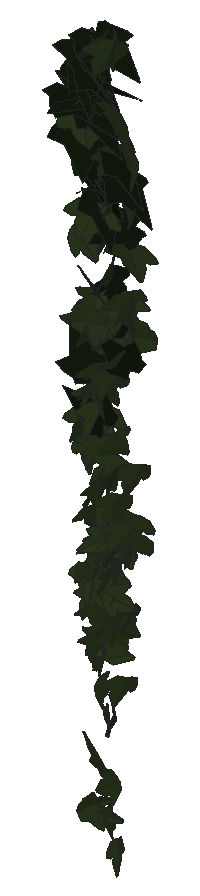
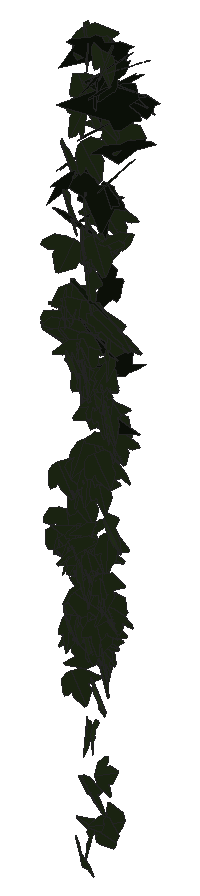
# SketchUp Ruby script. Lengths in inches.
U = 1.inch
M = Sketchup.active_model
def pt(a) = Geom::Point3d.new(a.map { |v| v * U })
def face(e, loops, mat)
  f = e.add_face(loops[0].map { |a| pt(a) })
  loops[1..].each { |l| e.add_face(l.map { |a| pt(a) }).erase! }
  f.material = f.back_material = mat if mat
  f
end
# faces: each face lists its corners as indices into pts; further lists are holes
def faces(e, pts, list, mat = nil) = list.each { |f| face(e, (f[0].is_a?(Array) ? f : [f]).map { |l| l.map { |i| pts[i] } }, mat) }
# xy, xz, yz: faces in a plane at the given z, y or x. An outline is a flat list of corners, or four numbers for a rectangle; further outlines are holes
def ring(l) = l.size == 4 ? [[l[0], l[1]], [l[2], l[1]], [l[2], l[3]], [l[0], l[3]]] : l.each_slice(2).to_a
def flat(e, list, mat, &to3) = list.each { |f| face(e, (f[0].is_a?(Array) ? f : [f]).map { |l| ring(l).map { |u, v| to3.(u, v) } }, mat) }
def xy(e, z, list, mat = nil) = flat(e, list, mat) { |x, y| [x, y, z] }
def xz(e, y, list, mat = nil) = flat(e, list, mat) { |x, z| [x, y, z] }
def yz(e, x, list, mat = nil) = flat(e, list, mat) { |y, z| [x, y, z] }
def lines(e, pts, list) = list.each { |a, b| e.add_line(pt(pts[a]), pt(pts[b])) }
# prism: a flat outline (further loops are holes) pulled along v
def prism(e, loops, v, mat = nil)
  f = face(e, loops, mat); d = Geom::Vector3d.new(v.map { |x| x * U })
  f.pushpull(f.normal.samedirection?(d) ? d.length : -d.length)
end
def box(e, o, s, mat = nil) = prism(e, [[o, [o[0] + s[0], o[1], o[2]], [o[0] + s[0], o[1] + s[1], o[2]], [o[0], o[1] + s[1], o[2]]]], [0, 0, s[2]], mat)
def at(x, y, z, deg = 0) = Geom::Transformation.translation(pt([x, y, z])) * Geom::Transformation.rotation(ORIGIN, Z_AXIS, deg.degrees)
def axes(o, x, y, z) = Geom::Transformation.new([*x, 0, *y, 0, *z, 0, *pt(o).to_a, 1])
def part(name) = M.definitions.add(name)
# library, detail: a bought-in or finely detailed component or shape, given as its bounding box
def library(name, o, s) = part(name).tap { |d| box(d.entities, o, s) }
def detail(e, o, s) = box(e.add_group.entities, o, s)
def put(e, d, t, mat = nil) = e.add_instance(d, t).tap { |i| i.material = mat if mat }
def group(e, t, mat = nil) = e.add_group.tap { |g| g.transformation = t; g.material = mat if mat }.entities
root = M.entities
M.materials.add("1026 AP 7946 SUNNY SIDE UP").color = [254, 231, 186]
M.materials.add("efeu1").color = [18, 25, 13]
M.materials.add("efeu2").color = [43, 57, 29]
c1 = part("ivyleaf_10")
p = [[0,0.5,-0.03],[-0.0625,2.02,-0.43],[-0.19,2.01,-0.46],[-0.54,1.05,-0.29],[-0.52,0.625,-0.18],[-0.83,0.76,-0.28],
  [-1.16,0.64,-0.33],[-1.15,0.33,-0.24],[-0.77,-0.39,0.02],[-0.3,-0.51,0.16],[0.04,-0.48,0.23],[-0.02,2.01,-0.4375],
  [-0.06,2.01,-0.43],[0.04,-0.49,0.23],[0.67,-0.49,0.14],[1.38,0.36,-0.2],[1.375,0.51,-0.24],[0.81,0.65,-0.19],
  [0.62,0.59,-0.15],[0.6,1.09,-0.28],[0.5,1.23,-0.31]]
faces(c1.entities,p,[[0,1,2,3,4,5,6,7,8,9,10],[11,12,0,13,14,15,16,17,18,19,20]],"efeu2")
c2 = part("ivyleaf_9")
p = [[1.54,2.16,1.25],[1.36,2.04,1.19],[-0.21,0.99,0.68],[-0.71,1.11,0.82],[-0.85,0.86,0.67],[-0.8,0.17,0.21],
  [-0.9,-0.01,0.1],[-0.67,-0.16,-0.02],[-0.08,-0.08,-0.05],[-0.03,-0.6,-0.4],[0.65,-0.88,-0.66],[0.83,-0.6,-0.49],
  [1.29,-0.42,-0.43],[1.8125,-0.07,-0.26],[1.21,0.44,0.15]]
faces(c2.entities,p,[[0,1,2,3,4,5,6,7,8,9,10,11,12,13,14]],"efeu1")
put(root,c1,axes([97.41,212.91,259.63],[0.10949,-0.19734,0.03462],[0.00095,-0.03655,-0.21548],[0.31507,0.06869,-0.01138]),"1026 AP 7946 SUNNY SIDE UP")
put(root,c2,axes([97.3125,212.78,265.79],[-0.1247,-0.23157,-0.03696],[0.03509,0.02884,-0.25171],[0.36648,-0.08156,0.01152]),"1026 AP 7946 SUNNY SIDE UP")
put(root,c1,axes([97.43,212.875,261.5],[0.0398,-0.22079,-0.03862],[-0.00634,0.03601,-0.22874],[0.35176,0.02563,0.00025]),"1026 AP 7946 SUNNY SIDE UP")
put(root,c2,axes([97.1,212.91,266.58],[0.33752,-0.03414,0.13387],[0.21069,0.03213,-0.21881],[0.01909,0.24896,0.0481]),"1026 AP 7946 SUNNY SIDE UP")
put(root,c2,axes([97.38,212.9,267.02],[-0.18909,-0.20027,0.10554],[0.00393,-0.11857,-0.23388],[0.35451,-0.10551,0.05889]),"1026 AP 7946 SUNNY SIDE UP")
put(root,c1,axes([97.36,212.92,258.26],[0.31557,-0.04478,0.0197],[0.02354,-0.02155,-0.21118],[0.07301,0.20047,-0.01706]),"1026 AP 7946 SUNNY SIDE UP")
put(root,c1,axes([97.43,212.97,261.54],[0.10388,-0.20513,-0.06291],[-0.00085,0.06254,-0.22088],[0.33602,0.06357,0.01889]),"1026 AP 7946 SUNNY SIDE UP")
put(root,c1,axes([97.42,212.91,259.36],[-0.09153,-0.1926,-0.0574],[0.03273,0.05075,-0.20692],[0.31308,-0.06161,0.00485]),"1026 AP 7946 SUNNY SIDE UP")
put(root,c2,axes([97.58,212.73,266.62],[-0.36277,-0.04896,0.03114],[-0.04029,-0.02881,-0.23387],[0.08849,-0.21383,0.02119]),"1026 AP 7946 SUNNY SIDE UP")
put(root,c1,axes([97.44,212.99,258.75],[-0.08302,-0.19748,-0.02475],[0.02284,0.0198,-0.21027],[0.31176,-0.05404,0.00882]),"1026 AP 7946 SUNNY SIDE UP")
put(root,c1,axes([97.43,212.82,262.5],[0.02247,-0.20885,-0.10627],[0.03565,0.10293,-0.2133],[0.3637,0.00282,0.02747]),"1026 AP 7946 SUNNY SIDE UP")
put(root,c1,axes([97.37,212.86,258.4],[-0.07173,-0.16061,-0.12519],[0.12446,0.0993,-0.16648],[0.29027,-0.08227,0.04044]),"1026 AP 7946 SUNNY SIDE UP")
put(root,c1,axes([97.58,212.9,262.92],[0.25928,-0.04659,-0.15665],[-0.22743,0.04621,-0.17621],[0.103,0.21931,0.00525]),"1026 AP 7946 SUNNY SIDE UP")
put(root,c1,axes([97.68,212.7,262.68],[0.13861,-0.05263,-0.2141],[-0.32312,0.06301,-0.10043],[0.13429,0.20595,-0.02066]),"1026 AP 7946 SUNNY SIDE UP")
put(root,c1,axes([97.35,212.73,266.0625],[0.3438,0.11325,0.03898],[0.0364,0.033,-0.2472],[-0.19786,0.20285,0.02225]),"1026 AP 7946 SUNNY SIDE UP")
put(root,c2,axes([97.35,212.87,266.79],[-0.0428,-0.25245,0.01228],[-0.00102,-0.01336,-0.26165],[0.3975,-0.02721,0.00065]),"1026 AP 7946 SUNNY SIDE UP")
put(root,c1,axes([97.45,212.8,260.98],[0.31657,0.07471,-0.04975],[-0.07101,-0.01833,-0.22133],[-0.12094,0.20632,-0.00027]),"1026 AP 7946 SUNNY SIDE UP")
put(root,c2,axes([97.31,212.85,265.34],[0.14624,-0.22144,-0.05789],[-0.03337,0.05067,-0.24714],[0.3572,0.09539,0.00062]),"1026 AP 7946 SUNNY SIDE UP")
put(root,c1,axes([97.44,212.9,267.3],[-0.14934,0.23434,-0.04559],[0.00982,-0.0466,-0.26049],[-0.37525,-0.09448,0.01132]),"1026 AP 7946 SUNNY SIDE UP")
put(root,c1,axes([97.41,212.6,264.15],[0.04409,0.21159,0.10297],[0.02227,0.09251,-0.22692],[-0.392,0.02906,-0.00131]),"1026 AP 7946 SUNNY SIDE UP")
put(root,c1,axes([97.55,212.9,267.33],[-0.01409,-0.25695,-0.01454],[-0.0099,0.01288,-0.2647],[0.40439,-0.00864,-0.00699]),"1026 AP 7946 SUNNY SIDE UP")
put(root,c1,axes([97.5,212.51,261.08],[0.03914,-0.19772,-0.1437],[0.04456,0.14053,-0.20081],[0.37684,0.00392,0.03867]),"1026 AP 7946 SUNNY SIDE UP")
put(root,c1,axes([97.5625,212.88,266.39],[-0.04874,-0.2407,0.06894],[-0.01791,-0.06738,-0.2504],[0.39301,-0.03292,-0.00286]),"1026 AP 7946 SUNNY SIDE UP")
put(root,c1,axes([97.53,212.99,258.68],[0.16959,-0.15565,-0.08188],[-0.01475,0.08711,-0.19046],[0.27379,0.1011,0.04046]),"1026 AP 7946 SUNNY SIDE UP")
put(root,c1,axes([97.51,212.82,258.01],[-0.0743,-0.16206,0.11907],[0.04999,-0.1243,-0.16558],[0.30983,-0.01881,0.05527]),"1026 AP 7946 SUNNY SIDE UP")
put(root,c2,axes([97.29,212.91,266.93],[0.20147,-0.21054,0.06703],[0.03813,-0.06273,-0.25399],[0.34496,0.1299,-0.01107]),"1026 AP 7946 SUNNY SIDE UP")
put(root,c1,axes([97.56,212.85,261.42],[-0.13936,-0.19211,0.07095],[0.00967,-0.07872,-0.21513],[0.32134,-0.08095,0.03724]),"1026 AP 7946 SUNNY SIDE UP")
put(root,c1,axes([97.55,212.91,261.82],[0.01366,-0.22215,0.00824],[0.00276,-0.0092,-0.22908],[0.3496,0.00875,0.00148]),"1026 AP 7946 SUNNY SIDE UP")
put(root,c2,axes([97.66,212.59,261.91],[-0.27229,-0.13499,0.08524],[0.09659,0.05868,0.22511],[-0.24952,0.17002,-0.00587]),"1026 AP 7946 SUNNY SIDE UP")
put(root,c2,axes([97.31,212.59,266.55],[-0.03922,-0.12421,-0.23356],[0.2185,0.18481,-0.11935],[0.34161,-0.13247,0.04953]),"1026 AP 7946 SUNNY SIDE UP")
put(root,c1,axes([97.41,212.76,260.57],[0.25607,-0.07791,0.12619],[0.1673,-0.06214,-0.18614],[0.15614,0.19435,-0.0075]),"1026 AP 7946 SUNNY SIDE UP")
put(root,c1,axes([97.52,212.82,262.03],[-0.02334,-0.15613,-0.17792],[0.09487,0.16366,-0.15762],[0.35251,-0.05438,0.03064]),"1026 AP 7946 SUNNY SIDE UP")
put(root,c1,axes([97.58,212.89,261.51],[-0.01832,-0.22004,-0.014],[0.01514,0.01183,-0.22674],[0.3462,-0.01216,0.00917]),"1026 AP 7946 SUNNY SIDE UP")
put(root,c1,axes([97.61,212.91,260.61],[-0.12848,-0.19291,0.07254],[0.00117,-0.07722,-0.21418],[0.32351,-0.07634,0.02958]),"1026 AP 7946 SUNNY SIDE UP")
put(root,c1,axes([97.56,212.96,261.79],[-0.2152,0.16719,-0.0641],[-0.00291,-0.08089,-0.21688],[-0.28102,-0.1272,0.05134]),"1026 AP 7946 SUNNY SIDE UP")
put(root,c1,axes([97.52,212.97,261.72],[0.02366,0.22064,0.04239],[0.0065,0.03971,-0.22759],[-0.3525,0.01554,-0.00135]),"1026 AP 7946 SUNNY SIDE UP")
put(root,c1,axes([97.61,212.95,264.16],[-0.13331,-0.21988,0.03712],[0.00593,-0.0413,-0.2423],[0.35063,-0.0829,0.01822]),"1026 AP 7946 SUNNY SIDE UP")
put(root,c2,axes([97.67,212.8125,265],[0.08033,0.21862,0.03514],[-0.02944,0.03424,-0.23761],[-0.37343,0.04433,0.02629]),"1026 AP 7946 SUNNY SIDE UP")
put(root,c1,axes([97.47,212.86,258.19],[0.11821,-0.08322,0.19101],[0.16892,-0.15214,-0.11581],[0.27207,0.13061,-0.01109]),"1026 AP 7946 SUNNY SIDE UP")
put(root,c2,axes([97.41,212.89,266.17],[0.09668,-0.23367,-0.07013],[0.03352,0.07377,-0.2454],[0.38065,0.05285,0.03942]),"1026 AP 7946 SUNNY SIDE UP")
put(root,c1,axes([97.61,212.7,264.58],[0.36555,0.05858,-0.05644],[-0.07833,-0.03335,-0.23846],[-0.10952,0.21936,-0.01784]),"1026 AP 7946 SUNNY SIDE UP")
put(root,c2,axes([97.87,212.55,261.12],[-0.08292,0.08042,0.23271],[-0.22145,0.17622,-0.09767],[-0.3043,-0.15015,0.00767]),"1026 AP 7946 SUNNY SIDE UP")
put(root,c1,axes([97.64,212.73,257.4],[0.07201,-0.19263,-0.06818],[-0.00886,0.06549,-0.20337],[0.31959,0.04522,0.00972]),"1026 AP 7946 SUNNY SIDE UP")
put(root,c1,axes([97.59,212.93,258.82],[0.07216,-0.17776,-0.09658],[0.05977,0.10113,-0.17972],[0.30955,0.02191,0.05722]),"1026 AP 7946 SUNNY SIDE UP")
put(root,c1,axes([97.79,212.61,255.32],[-0.11931,0.1029,-0.16854],[-0.17158,0.12301,0.1321],[0.25177,0.1326,0.01016]),"1026 AP 7946 SUNNY SIDE UP")
put(root,c1,axes([97.79,212.75,261.67],[-0.2762,0.07441,0.12444],[-0.19136,0.01847,-0.19462],[-0.11354,-0.21213,0.0253]),"1026 AP 7946 SUNNY SIDE UP")
put(root,c2,axes([97.56,212.61,263.4375],[0.28664,-0.07852,-0.11234],[-0.16486,0.03745,-0.19873],[0.14731,0.1947,-0.00381]),"1026 AP 7946 SUNNY SIDE UP")
put(root,c2,axes([97.49,212.7,267],[0.14589,-0.20592,-0.11857],[-0.04595,0.11143,-0.23135],[0.36717,0.09576,0.01816]),"1026 AP 7946 SUNNY SIDE UP")
put(root,c1,axes([97.85,212.97,258.31],[-0.16414,-0.0146,0.17824],[-0.23834,-0.09099,-0.1026],[0.13343,-0.1805,0.03598]),"1026 AP 7946 SUNNY SIDE UP")
put(root,c2,axes([97.74,212.74,264.91],[0.21274,0.00807,-0.19011],[-0.30146,-0.00646,-0.1345],[-0.01686,0.21733,0.0061]),"1026 AP 7946 SUNNY SIDE UP")
put(root,c1,axes([97.73,212.96,261.92],[-0.1121,-0.09395,0.19704],[-0.05348,-0.19463,-0.11238],[0.33154,-0.06316,0.04849]),"1026 AP 7946 SUNNY SIDE UP")
put(root,c1,axes([97.68,212.75,257.82],[-0.19725,-0.15829,-0.02047],[0.03648,0.00576,-0.20749],[0.248,-0.12674,0.01424]),"1026 AP 7946 SUNNY SIDE UP")
put(root,c2,axes([97.625,212.89,266.58],[-0.10205,0.03602,-0.22114],[0.25338,-0.14425,-0.07529],[-0.25109,-0.16021,0.01391]),"1026 AP 7946 SUNNY SIDE UP")
put(root,c1,axes([97.72,212.86,258.99],[-0.10465,-0.18621,0.07715],[0.0108,-0.08205,-0.20155],[0.31603,-0.05886,0.03244]),"1026 AP 7946 SUNNY SIDE UP")
put(root,c2,axes([97.92,212.77,262.52],[-0.08883,0.11267,0.1911],[-0.15128,0.15325,-0.13048],[-0.3225,-0.10292,0.00857]),"1026 AP 7946 SUNNY SIDE UP")
put(root,c1,axes([97.65,212.46,254.53],[0.01654,-0.03686,0.20898],[0.00873,0.20331,0.03891],[-0.3244,0.00359,0.0117]),"1026 AP 7946 SUNNY SIDE UP")
put(root,c2,axes([97.51,212.91,267.43],[0.00296,-0.1614,-0.20783],[0.111,0.19346,-0.15837],[0.38961,-0.05389,0.0467]),"1026 AP 7946 SUNNY SIDE UP")
put(root,c2,axes([97.91,212.95,263.35],[-0.26809,0.13856,0.00497],[-0.02341,-0.01143,-0.22428],[-0.2341,-0.15754,0.01674]),"1026 AP 7946 SUNNY SIDE UP")
put(root,c1,axes([97.82,212.81,259.06],[0.17051,0.06087,-0.1772],[-0.20914,-0.11118,-0.12732],[-0.19714,0.1706,-0.01819]),"1026 AP 7946 SUNNY SIDE UP")
put(root,c1,axes([97.7,212.8,264.6],[0.11828,-0.17126,0.12096],[-0.06084,0.10972,0.19934],[-0.34507,-0.07805,0.00632]),"1026 AP 7946 SUNNY SIDE UP")
put(root,c1,axes([97.74,212.93,263.55],[0.05868,-0.21859,-0.0867],[0.00256,0.08421,-0.22745],[0.3676,0.03431,0.01542]),"1026 AP 7946 SUNNY SIDE UP")
put(root,c1,axes([97.76,212.66,261.97],[-0.10125,-0.21109,0.01188],[0.00544,-0.01529,-0.23492],[0.35906,-0.05929,0.00691]),"1026 AP 7946 SUNNY SIDE UP")
put(root,c1,axes([97.78,212.63,257.15],[0.17861,-0.16079,-0.09818],[-0.05035,0.09206,-0.20072],[0.28882,0.11549,0.02572]),"1026 AP 7946 SUNNY SIDE UP")
put(root,c1,axes([97.79,212.73,257.51],[-0.03691,-0.18177,0.12349],[-0.01215,-0.12084,-0.1894],[0.34305,-0.02383,0.00658]),"1026 AP 7946 SUNNY SIDE UP")
put(root,c1,axes([97.83,212.68,260.72],[-0.16428,-0.1777,0.10909],[-0.04522,-0.10613,-0.21132],[0.32293,-0.10526,0.0259]),"1026 AP 7946 SUNNY SIDE UP")
put(root,c1,axes([97.78,212.89,262.43],[-0.04678,-0.21903,-0.0592],[0.02216,0.0548,-0.2273],[0.35487,-0.03229,0.00639]),"1026 AP 7946 SUNNY SIDE UP")
put(root,c2,axes([97.64,212.84,264.67],[0.00984,-0.24295,0.00446],[-0.00149,-0.00574,-0.2504],[0.38211,0.00623,-0.00109]),"1026 AP 7946 SUNNY SIDE UP")
put(root,c1,axes([97.8,212.96,264.18],[0.07175,-0.21792,-0.09008],[0.00702,0.08861,-0.22783],[0.36843,0.04075,0.02188]),"1026 AP 7946 SUNNY SIDE UP")
put(root,c1,axes([97.82,212.63,261.26],[0.26604,0.12851,-0.08672],[-0.13422,-0.03315,-0.21608],[-0.22198,0.17407,0.02672]),"1026 AP 7946 SUNNY SIDE UP")
put(root,c1,axes([97.8,212.96,264.23],[0.06275,-0.23228,-0.04256],[0.00372,0.04096,-0.24238],[0.37059,0.03892,0.00964]),"1026 AP 7946 SUNNY SIDE UP")
put(root,c1,axes([97.69,212.62,258.24],[0.0835,0.1887,0.09056],[0.04544,0.08204,-0.2014],[-0.32345,0.06024,-0.00492]),"1026 AP 7946 SUNNY SIDE UP")
put(root,c1,axes([97.83,212.63,257.45],[-0.10016,-0.20348,0.05319],[-0.01221,-0.05285,-0.2198],[0.33032,-0.06366,0.008]),"1026 AP 7946 SUNNY SIDE UP")
put(root,c1,axes([97.84,212.77,261.78],[-0.09258,-0.19838,0.08562],[-0.02731,-0.08267,-0.21357],[0.33779,-0.06105,0.0062]),"1026 AP 7946 SUNNY SIDE UP")
put(root,c1,axes([97.75,212.68,261.5],[-0.08862,0.2253,-0.00848],[-0.00334,-0.01033,-0.23927],[-0.35456,-0.05622,0.00437]),"1026 AP 7946 SUNNY SIDE UP")
put(root,c1,axes([97.8125,212.61,260.05],[-0.04668,-0.21549,-0.00384],[0.0094,0.0017,-0.22401],[0.33873,-0.02975,0.00569]),"1026 AP 7946 SUNNY SIDE UP")
put(root,c1,axes([97.87,212.81,267.37],[-0.13934,-0.21959,0.10245],[-0.02961,-0.10065,-0.24378],[0.3787,-0.08867,0.01863]),"1026 AP 7946 SUNNY SIDE UP")
put(root,c1,axes([97.83,212.89,265.57],[-0.04436,-0.23306,0.08243],[0.0102,-0.08254,-0.2418],[0.388,-0.02448,0.01578]),"1026 AP 7946 SUNNY SIDE UP")
put(root,c1,axes([97.83,212.99,258.84],[0.02232,-0.19895,-0.05579],[0.00079,0.05318,-0.20512],[0.32374,0.01358,0.00435]),"1026 AP 7946 SUNNY SIDE UP")
put(root,c1,axes([97.86,212.92,262.16],[0.07285,-0.19657,-0.10793],[-0.03446,0.10132,-0.20746],[0.34772,0.05123,0.00205]),"1026 AP 7946 SUNNY SIDE UP")
put(root,c1,axes([97.76,212.83,259.47],[0.09121,0.2028,0.00635],[0.01101,0.00321,-0.2172],[-0.31879,0.05813,-0.00568]),"1026 AP 7946 SUNNY SIDE UP")
put(root,c1,axes([97.91,212.65,255.99],[0.01237,0.02145,-0.20989],[-0.0782,0.19812,0.02066],[0.31269,0.0487,0.01347]),"1026 AP 7946 SUNNY SIDE UP")
put(root,c1,axes([97.6,212.67,254.4],[-0.06886,0.01492,0.20366],[0.31136,0.01139,0.04439],[-0.01246,0.20208,-0.01635]),"1026 AP 7946 SUNNY SIDE UP")
put(root,c1,axes([97.83,213.02,262.08],[0.1636,-0.18687,-0.0688],[0.018,0.07978,-0.21456],[0.31095,0.0937,0.04862]),"1026 AP 7946 SUNNY SIDE UP")
put(root,c1,axes([97.875,212.74,257.6],[0.02021,-0.20562,0.01507],[-0.00041,-0.01584,-0.21233],[0.32427,0.01279,-0.00121]),"1026 AP 7946 SUNNY SIDE UP")
put(root,c1,axes([97.875,212.83,264.8125],[0.06848,-0.22494,-0.08682],[0.01536,0.08595,-0.23419],[0.37669,0.03739,0.02533]),"1026 AP 7946 SUNNY SIDE UP")
put(root,c1,axes([97.87,212.83,258.6],[0.15253,-0.16189,-0.08309],[-0.00187,0.08995,-0.1891],[0.28374,0.08762,0.04342]),"1026 AP 7946 SUNNY SIDE UP")
put(root,c1,axes([97.93,212.64,254.375],[-0.08941,0.12408,0.15915],[-0.12263,0.13294,-0.13943],[-0.28549,-0.09596,0.01005]),"1026 AP 7946 SUNNY SIDE UP")
put(root,c1,axes([97.72,212.71,256.52],[0.05244,-0.1107,-0.17603],[0.1329,-0.1493,0.1162],[-0.29033,-0.08834,0.0214]),"1026 AP 7946 SUNNY SIDE UP")
put(root,c1,axes([97.87,212.79,260.24],[-0.04332,-0.2088,-0.05744],[0.0534,0.05013,-0.21498],[0.33511,-0.03498,0.02683]),"1026 AP 7946 SUNNY SIDE UP")
put(root,c1,axes([97.92,212.78,258.875],[0.05638,-0.20195,-0.05719],[-0.03362,0.05134,-0.21066],[0.32713,0.04008,-0.01179]),"1026 AP 7946 SUNNY SIDE UP")
put(root,c1,axes([97.9375,212.75,261.84],[-0.17051,-0.18632,0.06128],[-0.02546,-0.06043,-0.22185],[0.30699,-0.1085,0.01564]),"1026 AP 7946 SUNNY SIDE UP")
put(root,c1,axes([97.76,212.875,259.15],[-0.13001,-0.11003,-0.18776],[0.22287,0.11655,-0.13852],[0.24865,-0.162,0.02599]),"1026 AP 7946 SUNNY SIDE UP")
put(root,c1,axes([97.89,212.82,267.43],[0.13747,-0.23528,-0.06116],[0.03607,0.06945,-0.25407],[0.37933,0.07866,0.04632]),"1026 AP 7946 SUNNY SIDE UP")
put(root,c1,axes([97.875,212.92,260.73],[-0.05136,-0.18704,-0.10985],[0.08249,0.0966,-0.19248],[0.32749,-0.05366,0.03125]),"1026 AP 7946 SUNNY SIDE UP")
put(root,c1,axes([97.9375,212.73,256.11],[0.04953,-0.14205,-0.153],[-0.01105,0.14861,-0.1479],[0.32204,0.02694,0.01846]),"1026 AP 7946 SUNNY SIDE UP")
put(root,c1,axes([98.04,212.76,260.37],[-0.1548,-0.12408,0.16303],[-0.12127,-0.14027,-0.16283],[0.29297,-0.12363,0.01874]),"1026 AP 7946 SUNNY SIDE UP")
put(root,c1,axes([98.15,212.59,257.47],[0.01327,-0.00941,-0.20819],[-0.3178,0.0526,-0.01005],[0.08995,0.18725,-0.00482]),"1026 AP 7946 SUNNY SIDE UP")
put(root,c1,axes([97.91,212.98,262.39],[0.22963,-0.17405,-0.00578],[0.00123,0.00669,-0.23397],[0.27378,0.14596,0.0059]),"1026 AP 7946 SUNNY SIDE UP")
put(root,c1,axes([97.95,212.71,258.5625],[0.03988,-0.19174,0.07692],[0.00042,-0.0763,-0.19948],[0.32417,0.02369,-0.0092]),"1026 AP 7946 SUNNY SIDE UP")
put(root,c1,axes([98.1,212.9,259.05],[-0.13727,-0.06742,0.18753],[-0.15029,-0.15926,-0.1087],[0.26632,-0.12463,0.03532]),"1026 AP 7946 SUNNY SIDE UP")
put(root,c1,axes([98.07,212.58,255.07],[0.18202,-0.11849,-0.13385],[-0.14714,0.08924,-0.17009],[0.23318,0.14881,-0.00285]),"1026 AP 7946 SUNNY SIDE UP")
put(root,c1,axes([98,212.97,259.08],[0.13388,-0.18812,-0.02356],[-0.02783,0.0159,-0.2124],[0.29647,0.08644,-0.0093]),"1026 AP 7946 SUNNY SIDE UP")
put(root,c2,axes([98.18,212.91,264.4],[-0.35751,0.06628,0.01267],[-0.03184,-0.02333,-0.23481],[-0.10952,-0.20959,0.02689]),"1026 AP 7946 SUNNY SIDE UP")
put(root,c1,axes([97.92,212.95,259],[-0.30992,-0.03437,-0.05697],[0.09933,-0.06054,-0.19422],[0.02372,-0.1955,0.06887]),"1026 AP 7946 SUNNY SIDE UP")
put(root,c1,axes([97.99,212.8,257.77],[0.00782,-0.19425,0.06218],[0.01374,-0.06122,-0.20042],[0.32007,0.00737,0.00708]),"1026 AP 7946 SUNNY SIDE UP")
put(root,c1,axes([97.92,212.97,262.44],[0.11985,0.21567,0.00072],[-0.01486,0.00279,-0.23541],[-0.33879,0.07617,0.01058]),"1026 AP 7946 SUNNY SIDE UP")
put(root,c1,axes([97.89,212.94,263.07],[0.30606,0.12397,0.02178],[0.03214,0.00593,-0.23763],[-0.19493,0.19563,-0.00499]),"1026 AP 7946 SUNNY SIDE UP")
put(root,c1,axes([98.07,212.9375,262.73],[-0.09076,-0.11407,0.1954],[-0.05975,-0.18866,-0.12947],[0.34374,-0.06292,0.02908]),"1026 AP 7946 SUNNY SIDE UP")
put(root,c1,axes([97.87,212.68,257.1875],[0.24465,0.10311,-0.12166],[0.13884,0.08085,0.19208],[0.20454,-0.17821,0.01514]),"1026 AP 7946 SUNNY SIDE UP")
put(root,c1,axes([98.05,212.74,259.8],[-0.12799,-0.19434,0.06093],[-0.00991,-0.06245,-0.21667],[0.31977,-0.07972,0.01767]),"1026 AP 7946 SUNNY SIDE UP")
put(root,c1,axes([97.9,212.99,262.58],[0.32743,0.09125,0.02947],[0.04975,-0.00238,-0.23373],[-0.14164,0.2101,-0.01399]),"1026 AP 7946 SUNNY SIDE UP")
put(root,c1,axes([98.03,212.75,258.69],[0.16587,-0.17706,-0.06176],[-0.0227,0.05976,-0.21121],[0.29255,0.10502,0.01862]),"1026 AP 7946 SUNNY SIDE UP")
put(root,c1,axes([98.04,212.7,260.32],[0.06772,-0.21813,0.00597],[-0.00169,-0.00738,-0.22908],[0.34316,0.04301,-0.00231]),"1026 AP 7946 SUNNY SIDE UP")
put(root,c1,axes([97.97,212.83,259.29],[-0.08301,-0.15235,-0.14081],[0.12378,0.11424,-0.16286],[0.2961,-0.09047,0.0286]),"1026 AP 7946 SUNNY SIDE UP")
put(root,c1,axes([98.04,212.99,262.28],[0.07114,-0.21957,0.02655],[0.01068,-0.02619,-0.2311],[0.3477,0.04573,0.00167]),"1026 AP 7946 SUNNY SIDE UP")
put(root,c1,axes([98.07,212.95,262.19],[0.20995,-0.18065,-0.03719],[-0.02731,0.03076,-0.2312],[0.28807,0.13458,0.00518]),"1026 AP 7946 SUNNY SIDE UP")
put(root,c1,axes([98.14,212.83,259.24],[-0.15433,-0.15554,0.10857],[-0.05014,-0.10439,-0.18834],[0.29193,-0.10016,0.02505]),"1026 AP 7946 SUNNY SIDE UP")
put(root,c1,axes([98.15,212.54,266.4],[0.30341,-0.0741,-0.15025],[-0.1275,0.15191,-0.18969],[0.22273,0.1879,0.09609]),"1026 AP 7946 SUNNY SIDE UP")
put(root,c2,axes([97.91,212.85,265.52],[0.12843,-0.22925,-0.04548],[-0.0127,0.04259,-0.25038],[0.3665,0.08181,0.00726]),"1026 AP 7946 SUNNY SIDE UP")
put(root,c1,axes([98.0625,212.625,258.13],[0.02849,-0.1824,-0.10071],[0.05065,0.0984,-0.18438],[0.32066,0.00066,0.03807]),"1026 AP 7946 SUNNY SIDE UP")
put(root,c1,axes([98.09,212.9,263.16],[-0.17407,-0.20415,-0.03547],[0.05358,0.01922,-0.23819],[0.3208,-0.11398,0.02054]),"1026 AP 7946 SUNNY SIDE UP")
put(root,c1,axes([98.26,212.875,259.18],[-0.29813,-0.03963,0.11835],[-0.16781,-0.0484,-0.19854],[0.09209,-0.21646,0.02135]),"1026 AP 7946 SUNNY SIDE UP")
put(root,c1,axes([98.1,212.95,262.6875],[0.3416,0.05842,-0.05046],[-0.06773,-0.02921,-0.23129],[-0.09932,0.22085,-0.01584]),"1026 AP 7946 SUNNY SIDE UP")
put(root,c1,axes([98.11,212.91,257.81],[-0.05914,-0.19111,-0.06221],[0.04242,0.05495,-0.19973],[0.31176,-0.04373,0.01538]),"1026 AP 7946 SUNNY SIDE UP")
put(root,c1,axes([97.94,212.86,259.26],[0.18624,0.12402,0.14388],[0.15081,0.10056,-0.17608],[-0.25106,0.15241,0.00097]),"1026 AP 7946 SUNNY SIDE UP")
put(root,c1,axes([98.09,212.96,263.96],[-0.36056,-0.01147,-0.05262],[0.08217,-0.04284,-0.23233],[0.00267,-0.23097,0.04431]),"1026 AP 7946 SUNNY SIDE UP")
put(root,c1,axes([98.08,213.01,258.96],[-0.02869,0.10511,-0.18152],[0.00493,-0.17732,-0.10998],[-0.32337,-0.01203,0.01443]),"1026 AP 7946 SUNNY SIDE UP")
put(root,c2,axes([97.99,212.9,265.16],[0.08788,-0.21442,-0.13843],[-0.04252,0.13051,-0.22743],[0.39459,0.06181,0.00632]),"1026 AP 7946 SUNNY SIDE UP")
put(root,c1,axes([98.13,212.95,264.69],[0.19703,-0.2062,-0.01316],[0.00654,0.01609,-0.24818],[0.32468,0.12481,0.01299]),"1026 AP 7946 SUNNY SIDE UP")
put(root,c1,axes([98.09,212.75,266.03],[-0.24915,0.17505,-0.05859],[0.02947,-0.05943,-0.24402],[-0.31113,-0.14581,0.02381]),"1026 AP 7946 SUNNY SIDE UP")
put(root,c1,axes([98.18,212.9,265.43],[0.22508,-0.20896,-0.06232],[-0.04374,0.05281,-0.26054],[0.33874,0.14567,0.00777]),"1026 AP 7946 SUNNY SIDE UP")
put(root,c1,axes([98.2,212.69,256.78],[-0.11864,-0.18932,0.05647],[-0.00805,-0.05793,-0.20964],[0.31028,-0.07389,0.01615]),"1026 AP 7946 SUNNY SIDE UP")
put(root,c1,axes([98.12,212.77,259.84],[-0.03294,-0.00795,-0.23049],[-0.01161,-0.22452,0.00762],[-0.35175,0.00816,0.02133]),"1026 AP 7946 SUNNY SIDE UP")
put(root,c1,axes([98.17,212.82,259.03],[0.13556,-0.17937,-0.06193],[-0.00399,0.06385,-0.20311],[0.29693,0.08275,0.02554]),"1026 AP 7946 SUNNY SIDE UP")
put(root,c1,axes([98.14,212.8125,262.99],[-0.21312,0.19646,-0.01478],[-0.00395,-0.02049,-0.2456],[-0.30984,-0.13487,0.0133]),"1026 AP 7946 SUNNY SIDE UP")
put(root,c1,axes([98.23,212.86,259.48],[-0.32387,-0.03141,0.02775],[-0.03487,-0.0352,-0.2048],[0.0602,-0.18935,0.03066]),"1026 AP 7946 SUNNY SIDE UP")
put(root,c1,axes([98.17,212.8125,263.1],[-0.00239,-0.21566,-0.09801],[0.04622,0.09301,-0.21997],[0.36696,-0.01312,0.02706]),"1026 AP 7946 SUNNY SIDE UP")
put(root,c1,axes([98.23,212.96,260.27],[-0.12193,-0.19233,0.0605],[-0.01005,-0.06171,-0.21332],[0.31655,-0.07604,0.01653]),"1026 AP 7946 SUNNY SIDE UP")
put(root,c1,axes([98.05,212.7,253.95],[0.19196,-0.09522,0.14092],[0.16012,-0.09246,-0.15984],[0.20835,0.15879,-0.007]),"1026 AP 7946 SUNNY SIDE UP")
put(root,c1,axes([98.1,212.51,258.26],[0.03421,0.12283,0.16885],[0.04233,0.15411,-0.1311],[-0.33454,0.03206,0.00068]),"1026 AP 7946 SUNNY SIDE UP")
put(root,c1,axes([98.43,212.93,262.58],[-0.00662,-0.01156,-0.20648],[-0.32748,0.00784,0.00379],[0.01293,0.1926,-0.00985]),"1026 AP 7946 SUNNY SIDE UP")
put(root,c1,axes([98.22,212.65,262.36],[-0.02425,-0.2313,-0.01751],[0.01254,0.01518,-0.23862],[0.36432,-0.01592,0.00705]),"1026 AP 7946 SUNNY SIDE UP")
put(root,c1,axes([98.21,212.83,257.87],[0.08861,-0.19667,0.0011],[-0.00893,-0.0039,-0.21067],[0.30913,0.05626,-0.0064]),"1026 AP 7946 SUNNY SIDE UP")
put(root,c1,axes([98.16,212.68,257.69],[-0.06761,-0.12497,-0.16165],[0.09525,0.14414,-0.13513],[0.29978,-0.07398,0.00648]),"1026 AP 7946 SUNNY SIDE UP")
put(root,c2,axes([98.43,212.48,262.29],[-0.03656,0.07143,0.2122],[-0.20745,0.15694,-0.07293],[-0.28952,-0.12147,0.02546]),"1026 AP 7946 SUNNY SIDE UP")
